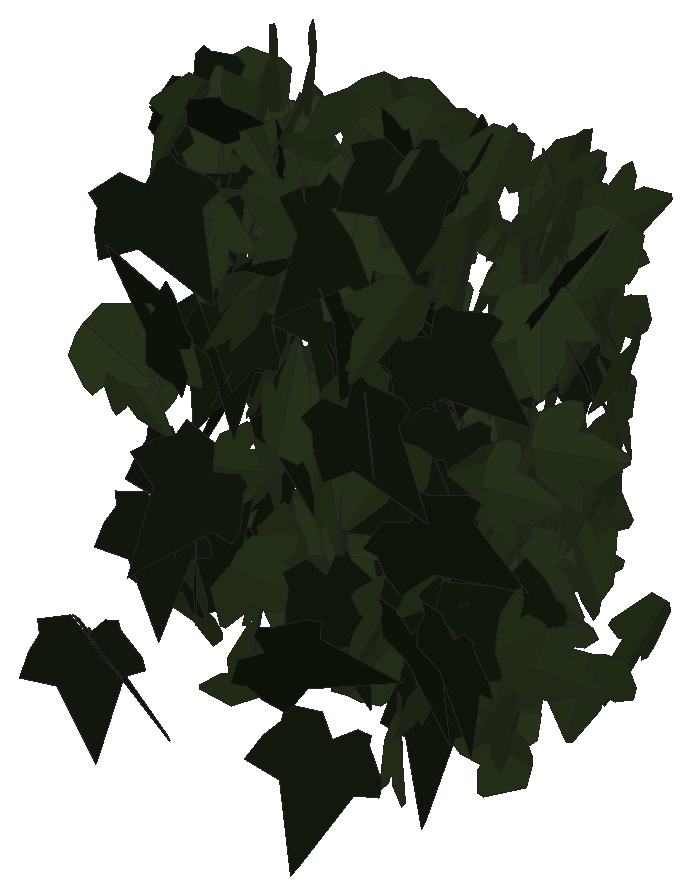
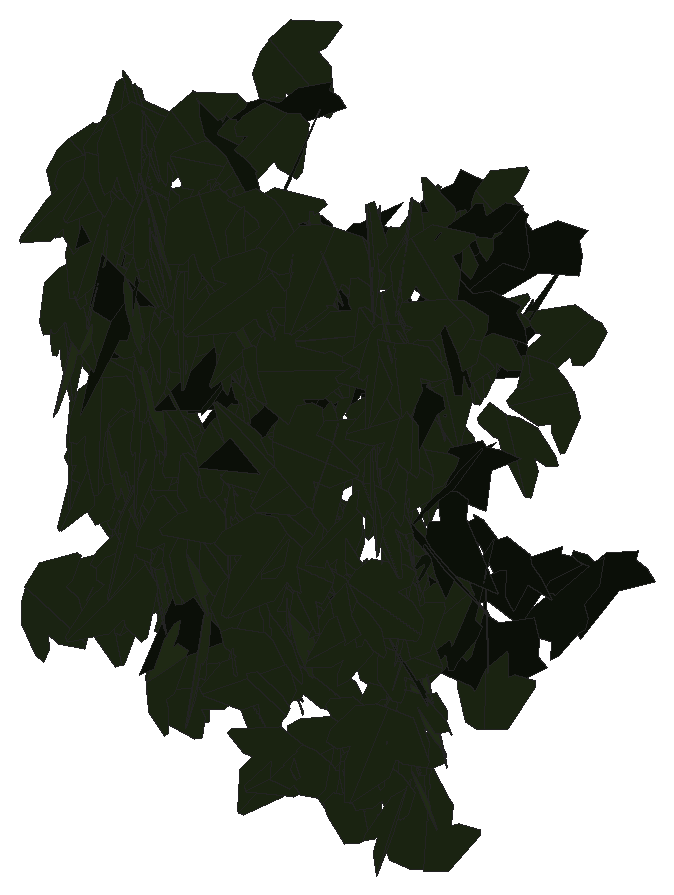
# SketchUp Ruby script. Lengths in inches.
U = 1.inch
M = Sketchup.active_model
def pt(a) = Geom::Point3d.new(a.map { |v| v * U })
def face(e, loops, mat)
  f = e.add_face(loops[0].map { |a| pt(a) })
  loops[1..].each { |l| e.add_face(l.map { |a| pt(a) }).erase! }
  f.material = f.back_material = mat if mat
  f
end
# faces: each face lists its corners as indices into pts; further lists are holes
def faces(e, pts, list, mat = nil) = list.each { |f| face(e, (f[0].is_a?(Array) ? f : [f]).map { |l| l.map { |i| pts[i] } }, mat) }
# xy, xz, yz: faces in a plane at the given z, y or x. An outline is a flat list of corners, or four numbers for a rectangle; further outlines are holes
def ring(l) = l.size == 4 ? [[l[0], l[1]], [l[2], l[1]], [l[2], l[3]], [l[0], l[3]]] : l.each_slice(2).to_a
def flat(e, list, mat, &to3) = list.each { |f| face(e, (f[0].is_a?(Array) ? f : [f]).map { |l| ring(l).map { |u, v| to3.(u, v) } }, mat) }
def xy(e, z, list, mat = nil) = flat(e, list, mat) { |x, y| [x, y, z] }
def xz(e, y, list, mat = nil) = flat(e, list, mat) { |x, z| [x, y, z] }
def yz(e, x, list, mat = nil) = flat(e, list, mat) { |y, z| [x, y, z] }
def lines(e, pts, list) = list.each { |a, b| e.add_line(pt(pts[a]), pt(pts[b])) }
# prism: a flat outline (further loops are holes) pulled along v
def prism(e, loops, v, mat = nil)
  f = face(e, loops, mat); d = Geom::Vector3d.new(v.map { |x| x * U })
  f.pushpull(f.normal.samedirection?(d) ? d.length : -d.length)
end
def box(e, o, s, mat = nil) = prism(e, [[o, [o[0] + s[0], o[1], o[2]], [o[0] + s[0], o[1] + s[1], o[2]], [o[0], o[1] + s[1], o[2]]]], [0, 0, s[2]], mat)
def at(x, y, z, deg = 0) = Geom::Transformation.translation(pt([x, y, z])) * Geom::Transformation.rotation(ORIGIN, Z_AXIS, deg.degrees)
def axes(o, x, y, z) = Geom::Transformation.new([*x, 0, *y, 0, *z, 0, *pt(o).to_a, 1])
def part(name) = M.definitions.add(name)
# library, detail: a bought-in or finely detailed component or shape, given as its bounding box
def library(name, o, s) = part(name).tap { |d| box(d.entities, o, s) }
def detail(e, o, s) = box(e.add_group.entities, o, s)
def put(e, d, t, mat = nil) = e.add_instance(d, t).tap { |i| i.material = mat if mat }
def group(e, t, mat = nil) = e.add_group.tap { |g| g.transformation = t; g.material = mat if mat }.entities
root = M.entities
M.materials.add("efeu1").color = [18, 25, 13]
M.materials.add("efeu2").color = [43, 57, 29]
c1 = part("ivyleaf_9")
p = [[1.54,2.16,1.25],[1.36,2.04,1.19],[-0.21,0.99,0.68],[-0.71,1.11,0.82],[-0.85,0.86,0.67],[-0.8,0.17,0.21],
  [-0.9,-0.01,0.1],[-0.67,-0.16,-0.02],[-0.08,-0.08,-0.05],[-0.03,-0.6,-0.4],[0.65,-0.88,-0.66],[0.83,-0.6,-0.49],
  [1.29,-0.42,-0.43],[1.8125,-0.07,-0.26],[1.21,0.44,0.15]]
faces(c1.entities,p,[[0,1,2,3,4,5,6,7,8,9,10,11,12,13,14]],"efeu1")
c2 = part("ivyleaf_10")
p = [[0,0.5,-0.03],[-0.0625,2.02,-0.43],[-0.19,2.01,-0.46],[-0.54,1.05,-0.29],[-0.52,0.625,-0.18],[-0.83,0.76,-0.28],
  [-1.16,0.64,-0.33],[-1.15,0.33,-0.24],[-0.77,-0.39,0.02],[-0.3,-0.51,0.16],[0.04,-0.48,0.23],[-0.02,2.01,-0.4375],
  [-0.06,2.01,-0.43],[0.04,-0.49,0.23],[0.67,-0.49,0.14],[1.38,0.36,-0.2],[1.375,0.51,-0.24],[0.81,0.65,-0.19],
  [0.62,0.59,-0.15],[0.6,1.09,-0.28],[0.5,1.23,-0.31]]
faces(c2.entities,p,[[0,1,2,3,4,5,6,7,8,9,10],[11,12,0,13,14,15,16,17,18,19,20]],"efeu2")
put(root,c1,axes([9.17,224.05,214.04],[0.13426,-0.23577,-0.35753],[-0.09997,0.33417,-0.27316],[0.43897,0.14822,0.04715]))
put(root,c2,axes([9.24,223.43,211.11],[0.46615,-0.05316,0.0105],[0.01092,-0.00051,-0.45228],[0.05741,0.43174,0.00076]))
put(root,c2,axes([9.23,225.49,212.94],[0.42615,0.1831,0.00128],[0.00474,-0.00653,-0.45233],[-0.19769,0.39453,-0.00808]))
put(root,c2,axes([9.27,225.45,207.26],[-0.10387,0.42195,0.04576],[-0.00867,0.0433,-0.45008],[-0.45809,-0.09649,-0.00185]))
put(root,c2,axes([9.33,223.75,214.05],[0.02415,-0.35025,0.26727],[0.03853,-0.25498,-0.36465],[0.46759,0.03911,0.01624]))
put(root,c1,axes([9.625,224.9,210.46],[-0.40097,0.19649,0.11756],[-0.1057,0.05671,-0.43684],[-0.22082,-0.38393,-0.00436]))
put(root,c2,axes([9.32,223.92,212.64],[-0.12434,-0.41878,0.02536],[0.06862,-0.0424,-0.44537],[0.44782,-0.10978,0.07529]))
put(root,c1,axes([9.16,224.26,213.17],[-0.21371,-0.23332,-0.32161],[0.2612,0.19686,-0.31541],[0.32683,-0.30989,0.04178]))
put(root,c2,axes([9.55,225.67,209.93],[0.17728,0.24306,-0.3341],[-0.34746,-0.12966,-0.273],[-0.26183,0.33665,0.13607]))
put(root,c2,axes([9.13,224.94,207.97],[-0.02965,-0.17998,-0.41087],[0.22092,-0.35452,0.15319],[-0.41356,-0.17648,0.11129]))
put(root,c1,axes([9.38,224.49,210.33],[-0.23041,0.1658,-0.35455],[0.24939,-0.2534,-0.27846],[-0.32469,-0.31229,0.03771]))
put(root,c2,axes([9.4,224.86,213.875],[-0.18721,-0.33137,0.23109],[0.02394,-0.2499,-0.36958],[0.43022,-0.13028,0.12113]))
put(root,c2,axes([9.32,225.5,211.44],[-0.39378,0.22473,-0.07906],[0.06642,-0.04508,-0.44539],[-0.24746,-0.36971,0.00625]))
put(root,c2,axes([9.5,224.1875,212.34],[0.04797,0.27211,0.41672],[-0.11252,-0.40188,0.27538],[0.48481,-0.1202,0.02268]))
put(root,c2,axes([9.51,224.79,209.52],[-0.13322,0.16794,0.39712],[-0.22639,0.31931,-0.21648],[-0.3895,-0.24303,-0.01]))
put(root,c2,axes([9.22,225.29,209.31],[-0.38063,0.02239,0.26416],[0.2688,-0.06401,0.36501],[0.05988,0.42968,0.04062]))
put(root,c2,axes([9.4,224.81,206.39],[-0.3092,-0.3194,-0.07533],[-0.04238,-0.06206,0.44591],[-0.35116,0.28872,0.01251]))
put(root,c1,axes([9.35,224.45,208.75],[0.29851,-0.33407,0.03644],[-0.01285,0.03561,0.45071],[-0.36254,-0.27633,0.01402]))
put(root,c2,axes([9.375,225.55,213.04],[0.01099,-0.40739,-0.15825],[0.07348,0.15183,-0.418],[0.46389,-0.0144,0.06996]))
put(root,c1,axes([9.32,223.58,209.72],[-0.35009,-0.09176,-0.28619],[0.29077,0.05843,-0.3501],[0.11661,-0.42118,0.01378]))
put(root,c1,axes([9.24,224.35,212.29],[-0.01028,0.28264,0.41232],[0.00326,-0.41236,0.28275],[0.49988,0.00851,0.00664]))
put(root,c2,axes([9.39,225.09,211.97],[0.04685,-0.10832,0.48587],[-0.07944,0.48014,0.1147],[-0.49142,-0.08794,0.02778]))
put(root,c2,axes([9.47,224.41,212.23],[-0.11992,-0.41782,0.05014],[-0.01362,-0.04654,-0.44961],[0.45403,-0.11175,-0.00024]))
put(root,c2,axes([9.39,225.3125,209.08],[-0.02553,-0.22466,0.38662],[0.07744,-0.36921,-0.2273],[0.46267,0.0494,0.05938]))
put(root,c2,axes([9.37,225.61,208.26],[-0.3357,-0.26445,-0.15659],[0.13636,0.08376,-0.42407],[0.29903,-0.33507,0.01758]))
put(root,c2,axes([9.3,224.32,209.27],[-0.08532,-0.16737,-0.40941],[0.20956,0.34275,-0.19205],[0.41172,-0.20913,0.0129]))
put(root,c2,axes([9.24,225.08,207.45],[0.24712,-0.20349,0.32132],[0.23558,-0.21922,-0.31816],[0.32272,0.31585,-0.01381]))
put(root,c2,axes([9.26,224.59,212.91],[0.10918,0.25113,0.35412],[0.12528,0.32022,-0.28143],[-0.43943,0.15369,0.00775]))
put(root,c2,axes([9.45,225.57,211.44],[0.15298,-0.38595,-0.14783],[-0.00667,0.14832,-0.42524],[0.44415,0.13516,0.04453]))
put(root,c2,axes([9.35,223.74,207.74],[-0.46831,0.04056,0.1704],[0.1629,-0.07795,0.46625],[0.06439,0.49222,0.0598]))
put(root,c2,axes([9.25,225.24,210.54],[0.22533,-0.24928,0.30062],[0.24733,-0.18179,-0.33496],[0.3298,0.30665,0.0458]))
put(root,c1,axes([9.42,224.4,211.0625],[-0.26986,-0.35546,-0.0218],[0.0128,0.01728,-0.45187],[0.38435,-0.25015,-0.00025]))
put(root,c2,axes([9.38,224.52,211.24],[0.04604,-0.22024,0.38761],[-0.01851,0.37335,0.23148],[-0.46717,-0.0365,0.02903]))
put(root,c1,axes([9.36,223.68,213.89],[0.37588,0.2587,-0.03557],[-0.02557,-0.02548,-0.45095],[-0.28066,0.34878,-0.00656]))
put(root,c1,axes([9.27,224.52,210.88],[0.05012,-0.42276,0.09501],[0.00283,-0.09161,-0.44225],[0.46711,0.04591,-0.00752]))
put(root,c2,axes([9.2,224.36,212.67],[0.09736,0.07088,-0.4364],[0.34577,0.27127,0.11919],[0.30278,-0.33259,0.00421]))
put(root,c2,axes([9.5,225.5625,211.06],[0.42123,-0.15778,-0.11493],[-0.10337,0.05782,-0.4372],[0.18054,0.40123,0.01781]))
put(root,c2,axes([9.46,224.03,213.3125],[0.13888,0.40062,-0.11484],[0.03148,0.10661,0.43755],[0.4477,-0.13177,0.00486]))
put(root,c2,axes([9.36,223.93,212.46],[0.45661,0.09135,0.04802],[0.03968,0.0477,-0.44804],[-0.10318,0.42262,0.04019]))
put(root,c1,axes([9.55,225.09,208.98],[-0.40007,0.11937,-0.20207],[0.19584,-0.07057,-0.40462],[-0.14934,-0.41231,0.01075]))
put(root,c2,axes([9.46,225.17,208.34],[0.46323,0.02487,-0.07084],[-0.07418,0.00828,-0.44664],[-0.02511,0.43421,0.01257]))
put(root,c2,axes([9.45,225.32,211.96],[-0.42649,0.16986,-0.06919],[0.0666,-0.02498,-0.44708],[-0.18542,-0.39968,-0.00146]))
put(root,c1,axes([9.375,223.17,209.14],[-0.09583,-0.41897,-0.07933],[0.01537,0.07496,-0.44539],[0.45967,-0.08985,-0.00165]))
put(root,c2,axes([9.34,222.19,211.78],[0.12877,0.28798,0.31558],[0.13339,0.27723,-0.3241],[-0.43167,0.17157,-0.00601]))
put(root,c2,axes([9.4375,225.07,208.22],[0.25243,0.36683,-0.00573],[0.0012,-0.00724,-0.45234],[-0.39622,0.23368,-0.00502]))
put(root,c2,axes([9.26,222.64,211.1875],[-0.24997,0.05642,-0.37853],[0.35206,-0.16872,-0.24278],[-0.18516,-0.39696,0.04939]))
put(root,c2,axes([9.56,225.19,213.1875],[0.17855,-0.40216,-0.01308],[-0.00422,0.01199,-0.45221],[0.43453,0.16537,0.00098]))
put(root,c2,axes([9.45,225.31,211.9375],[-0.43379,0.07735,-0.15394],[0.15104,-0.05497,-0.42455],[-0.0986,-0.42452,0.02692]))
put(root,c2,axes([9.45,225.16,207.8],[0.33395,0.30555,0.01637],[0.01216,0.01099,-0.4521],[-0.33021,0.30942,-0.0001]))
put(root,c2,axes([9.61,224.47,212.32],[0.20966,-0.38427,-0.06475],[-0.03794,0.052,-0.44767],[0.41871,0.19712,-0.00814]))
put(root,c1,axes([9.39,223.58,208.13],[-0.21274,-0.03123,0.40205],[0.41821,-0.04025,0.20182],[0.02359,0.43201,0.04787]))
put(root,c1,axes([9.375,223.75,208.94],[-0.05298,-0.02352,-0.44885],[0.44437,-0.13557,-0.04096],[-0.14296,-0.41267,0.03903]))
put(root,c1,axes([9.4,222.9375,213.29],[-0.05157,-0.31318,-0.38634],[0.11431,0.37055,-0.31564],[0.48402,-0.12088,0.03338]))
put(root,c2,axes([9.65,224.42,211.36],[-0.02962,-0.49129,-0.08806],[0.01275,0.08745,-0.49213],[0.49896,-0.0314,0.00734]))
put(root,c2,axes([9.63,224.91,210.34],[0.02736,-0.40702,-0.15743],[0.02014,0.15252,-0.42324],[0.46857,0.01721,0.02738]))
put(root,c2,axes([9.64,224.71,214.125],[0.17981,-0.36393,-0.29192],[-0.01136,0.30935,-0.39265],[0.46641,0.14784,0.10298]))
put(root,c2,axes([9.28,225.08,211.34],[-0.03612,0.00945,-0.45095],[0.39052,-0.23955,-0.03443],[-0.25866,-0.36298,0.01098]))
put(root,c2,axes([9.54,225.16,208.49],[-0.20583,0.26462,0.2994],[0.18509,-0.23133,0.33914],[0.37959,0.25629,-0.00302]))
put(root,c2,axes([9.46,225.1,212.49],[0.39764,0.20222,-0.2258],[0.18967,0.12455,0.44555],[0.23645,-0.43999,0.02234]))
put(root,c1,axes([9.35,224.9,212.23],[0.48622,-0.10323,0.05416],[0.05292,-0.01154,-0.49706],[0.10387,0.48909,-0.0003]))
put(root,c2,axes([9.31,225.28,210.99],[0.13091,-0.12269,0.4667],[0.44463,-0.15725,-0.16606],[0.18752,0.4585,0.06793]))
put(root,c2,axes([9.72,225.48,209.33],[0.04662,-0.04156,0.49608],[-0.12252,0.48197,0.05189],[-0.48251,-0.12639,0.03476]))
put(root,c1,axes([9.46,225.03,209.66],[0.23224,-0.37535,0.04759],[0.02647,-0.0387,-0.44989],[0.40752,0.21642,0.0021]))
put(root,c1,axes([9.84,222.86,211.57],[0.07403,-0.4705,0.15216],[-0.02373,0.1503,0.47629],[-0.49392,-0.07774,-0.00008]))
put(root,c1,axes([9.62,221.61,208.42],[-0.15044,-0.37027,-0.18814],[0.05184,0.17508,-0.41112],[0.44203,-0.14655,-0.01581]))
put(root,c2,axes([9.47,225.43,207.56],[0.32307,0.0626,0.32194],[0.31939,0.09412,-0.317],[-0.11971,0.42006,0.02305]))
put(root,c2,axes([9.53,225.81,209.78],[0.37364,-0.07058,0.26423],[0.26841,-0.0528,-0.36721],[0.09519,0.42597,-0.00174]))
put(root,c1,axes([9.46,221.98,208.19],[0.34901,-0.26872,0.11669],[0.09702,-0.06743,-0.43706],[0.29915,0.33536,0.00562]))
put(root,c2,axes([10.125,224.63,212.37],[-0.16838,-0.09001,-0.46211],[-0.41499,-0.2034,0.19082],[-0.22234,0.4478,-0.00621]))
put(root,c2,axes([9.6875,225.48,208.07],[-0.36731,0.1028,-0.26102],[0.22296,-0.16293,-0.36035],[-0.18996,-0.39001,0.08174]))
put(root,c2,axes([9.64,225.22,211.54],[0.10424,-0.25481,0.41738],[0.3017,-0.30234,-0.25993],[0.38485,0.30604,0.09072]))
put(root,c2,axes([9.49,224.17,213.78],[0.23592,-0.00784,0.44077],[0.44084,0.00453,-0.23588],[-0.0003,0.49992,0.00905]))
put(root,c2,axes([9.91,225.08,214.125],[0.23244,-0.39917,-0.1914],[-0.03567,0.19859,-0.45748],[0.44125,0.22633,0.06384]))
put(root,c1,axes([9.79,224.88,212.49],[-0.03425,-0.01446,0.49862],[0.01013,-0.49971,-0.01379],[0.49872,0.00916,0.03452]))
put(root,c2,axes([9.97,225.32,210.52],[0.08143,-0.01875,-0.49297],[0.03997,0.49825,-0.01234],[0.4917,-0.0374,0.08265]))
put(root,c2,axes([9.9,225.29,206.83],[0.09448,-0.48658,-0.06567],[0.022,-0.06262,0.49558],[-0.4905,-0.09653,0.00958]))
put(root,c2,axes([9.77,225.34,211.58],[0.31412,0.21991,0.2467],[0.20348,0.14413,-0.37921],[-0.28397,0.34654,0.00116]))
put(root,c2,axes([9.7,225.1,209.41],[0.15077,-0.07794,-0.47031],[0.46048,-0.10389,0.16483],[-0.12341,-0.48284,0.04045]))
put(root,c2,axes([9.79,225.08,212.85],[0.12007,-0.05897,0.43305],[0.32772,0.30946,-0.03869],[-0.31448,0.29997,0.12503]))
put(root,c1,axes([9.88,224.58,211.93],[-0.18931,-0.39806,0.00711],[0.42466,-0.17426,-0.06776],[0.06735,-0.02007,0.44724]))
put(root,c2,axes([10.49,225.74,211.47],[-0.00597,0.02453,-0.49936],[-0.4709,0.16752,0.01386],[0.16799,0.47046,0.0211]))
put(root,c2,axes([10.12,224.44,208.24],[-0.48238,-0.12794,0.03069],[0.04198,-0.03915,0.49669],[-0.12469,0.48177,0.04851]))
put(root,c2,axes([10.43,225.58,209.89],[-0.09571,0.12749,-0.47391],[-0.32239,0.3477,0.15865],[0.37,0.33594,0.01564]))
put(root,c2,axes([10.16,225.54,211.59],[-0.26854,0.39612,-0.14481],[0.08066,-0.12027,-0.47857],[-0.41398,-0.2804,0.00069]))
put(root,c2,axes([10.63,225.49,210.41],[0.24965,-0.03764,-0.43158],[-0.42662,0.0652,-0.25247],[0.07528,0.4943,0.00044]))
put(root,c2,axes([10.8125,225.62,212.27],[-0.12604,0.12606,-0.46714],[-0.48289,-0.00237,0.12965],[0.03048,0.48384,0.12235]))
put(root,c2,axes([10.43,225.24,213.74],[-0.3137,-0.33861,-0.19217],[0.14942,0.12319,-0.46098],[0.35953,-0.34665,0.0239]))
put(root,c2,axes([10.43,224.83,209.27],[-0.06239,0.49353,-0.05039],[0.00544,-0.05011,-0.49745],[-0.49606,-0.06262,0.00089]))
put(root,c2,axes([10.59,225.35,212.8125],[0.46416,0.10744,-0.1517],[-0.15022,-0.02358,-0.47632],[-0.1095,0.48775,0.01039]))
put(root,c2,axes([10.33,225.58,211.2],[-0.37182,0.03772,-0.33216],[0.32998,-0.03811,-0.37371],[-0.05351,-0.49712,0.00344]))
put(root,c2,axes([10.58,223.92,212.93],[-0.0979,0.34101,0.35232],[0.0733,-0.34505,0.35435],[0.48481,0.12103,0.01757]))
put(root,c2,axes([10.82,225.375,211.24],[0.31679,-0.12792,-0.36507],[-0.3398,0.1335,-0.34164],[0.18488,0.46456,-0.00235]))
put(root,c2,axes([10.45,223.31,208.81],[-0.17558,-0.24536,-0.39871],[0.27437,0.29111,-0.29996],[0.37933,-0.32412,0.03241]))
put(root,c2,axes([10.42,225.18,207.42],[-0.11155,-0.11661,-0.47324],[0.31749,0.35097,-0.16131],[0.36981,-0.33649,-0.00426]))
put(root,c2,axes([10.51,224.875,209.91],[0.02874,0.04497,0.49714],[0.06406,0.49352,-0.04834],[-0.49505,0.06647,0.0226]))
put(root,c2,axes([10.62,224.32,212.66],[-0.33267,0.28023,0.24658],[0.17059,-0.17964,0.43431],[0.332,0.3731,0.02392]))
put(root,c2,axes([10.86,224.3,211.63],[0.09859,-0.14269,0.46896],[-0.27671,0.37864,0.17338],[-0.40461,-0.29372,-0.00431]))
put(root,c2,axes([10.65,223.71,210.43],[0.48147,-0.13432,0.012],[-0.00983,0.00942,0.49981],[-0.13449,-0.48153,0.00643]))
put(root,c2,axes([10.91,225.05,208.29],[0.34712,0.10055,-0.34554],[-0.33035,-0.10137,-0.36137],[-0.14273,0.47918,-0.00394]))
put(root,c2,axes([10.57,225.52,209.16],[0.18764,-0.26669,0.37903],[0.23791,-0.2955,-0.3257],[0.39773,0.30258,0.016]))
put(root,c2,axes([10.69,225.01,213.57],[0.35609,-0.31025,0.16417],[0.117,-0.11556,-0.47218],[0.33093,0.37469,-0.0097]))
put(root,c2,axes([10.5625,225.68,207.52],[0.32362,0.23482,0.30022],[0.23426,0.18813,-0.39966],[-0.30066,0.39933,0.01174]))
put(root,c2,axes([10.83,225.59,210.05],[-0.40981,-0.16239,-0.23598],[0.21502,0.09777,-0.44069],[0.18927,-0.46268,-0.0103]))
put(root,c1,axes([11,221.98,210.77],[-0.26137,-0.38705,0.17853],[-0.09975,-0.14807,-0.46704],[0.41441,-0.27976,0.00018]))
put(root,c2,axes([10.75,224.63,209.21],[-0.03918,0.04455,-0.49647],[0.18716,-0.46025,-0.05607],[-0.46199,-0.19023,0.01939]))
put(root,c2,axes([11.19,225.57,207.99],[0.32489,-0.17434,-0.33772],[-0.30044,0.1543,-0.36868],[0.23277,0.44249,-0.0045]))
put(root,c2,axes([10.93,225.43,211.96],[-0.00355,-0.44485,-0.22825],[0.06456,-0.22676,0.44092],[-0.4958,-0.02634,0.05905]))
put(root,c2,axes([10.86,225.6,209],[0.40559,-0.19217,0.22039],[0.20865,-0.07381,-0.44835],[0.20485,0.45566,0.02032]))
put(root,c2,axes([11.12,225.07,212.91],[0.07562,-0.44922,0.20612],[0.01793,-0.20589,-0.45529],[0.49392,0.07625,-0.01503]))
put(root,c2,axes([11.04,224.83,212.36],[-0.35903,-0.19573,-0.28773],[0.25065,0.14133,-0.4089],[0.2414,-0.43785,-0.00336]))
put(root,c1,axes([11.03,224.71,211.04],[0.23785,0.20645,0.38834],[0.26531,0.28476,-0.31388],[-0.35077,0.35537,0.02592]))
put(root,c1,axes([11.21,224.09,212.93],[-0.182,-0.37966,0.26969],[-0.09115,-0.25492,-0.42037],[0.45669,-0.20218,0.02358]))
put(root,c2,axes([10.9375,225.625,208.45],[-0.29165,0.05766,-0.40201],[0.39623,-0.06821,-0.29724],[-0.08912,-0.49196,-0.00591]))
put(root,c2,axes([11.08,225.43,213.9],[-0.42164,0.12855,-0.236],[0.22025,-0.08632,-0.4405],[-0.15399,-0.47542,0.01617]))
put(root,c2,axes([10.95,225.48,210.87],[0.37572,-0.02833,-0.32868],[0.32979,0.01939,0.37532],[-0.00852,-0.49882,0.03326]))
put(root,c2,axes([11.34,225.23,213.78],[-0.22783,-0.36848,0.24963],[-0.03747,-0.26357,-0.42324],[0.4435,-0.21156,0.09249]))
put(root,c2,axes([11.09,225.52,213.24],[-0.18141,-0.20163,-0.42004],[0.31099,0.28326,-0.27028],[0.34695,-0.35932,0.02263]))
put(root,c1,axes([11.1,223.89,208.67],[0.13053,-0.44108,-0.196],[-0.05949,0.18679,-0.45997],[0.47898,0.14339,-0.00371]))
put(root,c2,axes([11.28,224.06,212.91],[0.46648,0.16986,-0.05953],[-0.05741,-0.01632,-0.49642],[-0.17059,0.46998,0.00428]))
put(root,c2,axes([11.3,225.09,212.54],[0.00604,0.29082,0.40668],[0.01089,0.40654,-0.29088],[-0.49984,0.01237,-0.00142]))
put(root,c1,axes([11.35,224.03,212.125],[-0.30908,-0.35942,-0.15901],[0.10179,0.12219,-0.47404],[0.37962,-0.3254,-0.00236]))
put(root,c2,axes([11.66,224.74,209.22],[0.30393,0.0049,-0.39699],[-0.39698,0.01081,-0.30379],[0.00561,0.49986,0.01046]))
put(root,c2,axes([11.375,225.37,208.57],[-0.0278,-0.17828,0.46631],[0.10609,-0.45847,-0.16896],[0.48782,0.08954,0.06332]))
put(root,c2,axes([11.69,225.05,208.92],[-0.21177,-0.25999,0.37089],[-0.20919,-0.307,-0.33465],[0.40174,-0.29691,0.02125]))
put(root,c2,axes([11.49,224.8,213.24],[0.15129,-0.46438,0.10706],[0.02737,-0.10367,-0.48837],[0.47578,0.15363,-0.00595]))
put(root,c2,axes([11.59,224.33,208.51],[0.13207,-0.40388,-0.26351],[-0.08229,0.25033,-0.42493],[0.47517,0.1556,-0.00035]))
put(root,c1,axes([11.32,224.62,211.47],[0.48962,-0.06341,-0.07904],[-0.07776,0.01499,-0.49369],[0.06498,0.49574,0.00482]))
put(root,c2,axes([11.56,225.01,211.22],[-0.07741,-0.39665,0.29441],[0.06444,-0.30356,-0.39204],[0.48975,-0.02275,0.09812]))
put(root,c2,axes([11.64,224.95,213.21],[-0.19961,-0.45754,0.0286],[-0.00949,-0.02707,-0.49918],[0.45833,-0.19982,0.00212]))
put(root,c1,axes([11.18,224.1,211.75],[0.08577,-0.11271,-0.47952],[0.42953,0.25539,0.0168],[0.24114,-0.41482,0.14063]))
put(root,c1,axes([11.8,224.88,213.08],[0.00383,0.01855,-0.49964],[-0.15317,-0.47559,-0.01884],[-0.47595,0.1532,0.00204]))
put(root,c1,axes([11.35,224.14,211.38],[0.27107,-0.41147,-0.08492],[-0.03858,0.07625,-0.49264],[0.41837,0.27363,0.00959]))
put(root,c1,axes([11.41,223.98,211.84],[0.04236,-0.31391,0.38687],[0.04032,-0.38483,-0.31667],[0.49657,0.05803,-0.00729]))
put(root,c2,axes([11.46,225.49,212.86],[0.17314,-0.23227,0.40752],[0.24742,-0.32383,-0.28969],[0.39851,0.30197,0.0028]))
put(root,c2,axes([11.73,225.4,210.95],[-0.05345,-0.43868,0.23389],[-0.01759,-0.23342,-0.44182],[0.49682,-0.05546,0.00952]))
put(root,c2,axes([11.78,225.19,210.77],[-0.145,-0.47265,0.07468],[-0.01768,-0.07269,-0.49437],[0.47819,-0.14601,0.00437]))
put(root,c2,axes([11.97,225.47,213.7],[-0.42074,-0.11229,0.2457],[-0.23682,-0.06547,-0.43546],[0.12997,-0.48281,0.00191]))
put(root,c2,axes([11.8125,225.23,210.31],[0.26014,-0.34554,-0.25085],[-0.07334,0.25322,-0.42485],[0.42065,0.25784,0.08107]))
put(root,c1,axes([11.67,224.6,213.47],[-0.10576,-0.09037,0.48026],[-0.03745,-0.48843,-0.10015],[0.48725,-0.05715,0.09654]))
put(root,c2,axes([11.65,223.87,207.65],[-0.09201,-0.39968,0.28599],[0.06715,0.27801,0.41012],[-0.48685,0.11388,0.00252]))
put(root,c2,axes([11.8,225.15,212.54],[0.05138,-0.49728,-0.00839],[0.00092,0.00853,-0.49993],[0.49735,0.05135,0.00179]))
put(root,c2,axes([11.79,223.44,211.64],[-0.14255,-0.35463,-0.32236],[0.10494,0.30506,-0.38201],[0.46762,-0.17657,-0.01254]))
put(root,c2,axes([11.87,225.57,208.49],[0.22819,-0.27831,-0.34709],[-0.0431,0.37442,-0.32856],[0.4428,0.17987,0.14689]))
put(root,c2,axes([11.73,225.19,212.66],[-0.03077,-0.12962,-0.48193],[0.12547,-0.46934,0.11822],[-0.48302,-0.11365,0.06141]))
put(root,c2,axes([11.72,225.38,209.99],[0.35171,0.258,-0.24441],[0.19959,0.14112,0.43617],[0.29405,-0.40438,-0.00372]))
put(root,c2,axes([11.56,225.27,211.66],[0.07929,-0.11117,0.48099],[0.44073,-0.20355,-0.1197],[0.22242,0.44296,0.06572]))
put(root,c2,axes([11.84,223.97,208.62],[0.06993,-0.30339,0.39123],[0.12235,-0.37227,-0.31055],[0.47973,0.13917,0.02217]))
put(root,c1,axes([11.62,224.3,210.49],[0.35236,-0.15617,-0.31852],[0.29079,-0.12999,0.38542],[-0.20319,-0.45685,-0.00078]))
put(root,c2,axes([11.85,225.16,212.15],[0.07726,-0.35066,0.34795],[0.20694,-0.29681,-0.34508],[0.44856,0.19733,0.09927]))
put(root,c1,axes([11.68,224.61,211.66],[0.44505,0.0815,0.21281],[0.20734,0.04892,-0.45235],[-0.09456,0.49088,0.00975]))
put(root,c2,axes([11.78,225.12,210.61],[0.30916,-0.21197,0.3309],[0.29076,-0.15983,-0.37405],[0.26435,0.4237,0.02444]))
put(root,c2,axes([12.28,223.53,210.75],[-0.26967,-0.32954,0.26207],[-0.13271,-0.22883,-0.42429],[0.39959,-0.29839,0.03595]))
put(root,c1,axes([12.09,222.68,207.54],[-0.30713,-0.38365,-0.0921],[0.05554,0.07352,-0.49144],[0.39063,-0.3121,-0.00254]))
put(root,c2,axes([11.99,224.88,213.37],[0.12384,0.41835,0.24422],[0.0674,0.23474,-0.43629],[-0.47971,0.14098,0.00175]))
put(root,c2,axes([12.26,225.1,209.35],[-0.1516,-0.40234,0.25522],[-0.08149,-0.24199,-0.42988],[0.46945,-0.17193,0.0078]))
put(root,c2,axes([12.52,224.65,208.75],[0.13939,0.02532,-0.47951],[-0.47741,0.06086,-0.13557],[0.0515,0.49564,0.04114]))
put(root,c1,axes([12.01,223.45,211.09],[-0.05222,0.06655,0.49279],[0.05695,-0.49144,0.0724],[0.49399,0.06369,0.04375]))
put(root,c1,axes([12.06,224.125,210.08],[-0.23417,-0.31285,-0.31192],[0.17788,0.25638,-0.39068],[0.40438,-0.29394,-0.00878]))
put(root,c2,axes([12.26,224.41,213.2],[0.20028,-0.45497,-0.05378],[-0.01744,0.05108,-0.49708],[0.4578,0.20098,0.00459]))
put(root,c1,axes([12.02,225.01,211.43],[-0.00212,-0.37618,0.32937],[0.13838,-0.31695,-0.3611],[0.48047,0.08963,0.10545]))
put(root,c2,axes([12.07,225.48,209.36],[0.22465,-0.25263,0.36839],[0.25708,-0.2641,-0.33788],[0.3653,0.34122,0.01123]))
put(root,c1,axes([12.21,224.7,210.49],[-0.09155,-0.48885,0.05146],[-0.00883,-0.0507,-0.49734],[0.49147,-0.09197,0.00065]))
put(root,c2,axes([12.4,225.21,212.46],[0.10986,-0.44479,-0.20023],[-0.01352,0.20239,-0.45701],[0.48759,0.10583,0.03244]))
put(root,c2,axes([12.65,225.39,207.65],[-0.18232,0.28434,-0.36866],[-0.26219,0.26446,0.33364],[0.38473,0.31498,0.05267]))
put(root,c2,axes([12.11,223.77,207.25],[0.15267,-0.07313,0.47047],[0.3987,-0.25042,-0.16831],[0.26025,0.42655,-0.01815]))
put(root,c1,axes([12.71,224.17,214.02],[-0.25449,0.39274,0.17604],[-0.09466,0.14843,-0.46798],[-0.41985,-0.27152,-0.0012]))
put(root,c1,axes([12.28,223.74,214.26],[-0.07865,-0.46045,-0.17834],[0.06328,0.1697,-0.46605],[0.4897,-0.09588,0.03158]))
put(root,c2,axes([12.48,223.92,207.9],[-0.02671,-0.41341,-0.27997],[0.00815,0.27997,-0.41419],[0.49922,-0.02669,-0.00822]))
put(root,c2,axes([12.31,223.72,213.98],[-0.08821,-0.30097,-0.3894],[0.23854,0.31989,-0.30128],[0.43048,-0.23893,0.08715]))
put(root,c2,axes([12.48,224.75,213.25],[0.1535,-0.47388,-0.0433],[-0.01326,0.04122,-0.49812],[0.47567,0.15407,0.00009]))
put(root,c2,axes([12.51,225.02,209.59],[-0.34329,-0.35998,-0.05065],[0.03445,0.03714,-0.49743],[0.36189,-0.34501,-0.0007]))
put(root,c1,axes([12.49,224.09,208.66],[-0.40632,-0.04997,0.28707],[0.28424,0.04043,0.40935],[-0.06412,0.49585,-0.00445]))
put(root,c1,axes([12.18,221.55,209.17],[0.0625,0.1625,-0.46871],[0.19848,0.42476,0.17373],[0.45464,-0.20778,-0.01142]))
put(root,c1,axes([12.41,224.07,207.68],[-0.35453,-0.08631,-0.34185],[0.33525,0.06755,-0.36475],[0.10915,-0.48784,0.00997]))
put(root,c2,axes([12.74,225.19,211.41],[0.06546,0.14434,0.47422],[-0.23123,-0.41421,0.15799],[0.43846,-0.23999,0.01253]))
put(root,c2,axes([12.87,224.9,207.24],[-0.0307,-0.02212,-0.49857],[-0.46352,-0.18385,0.0367],[-0.18495,0.46445,-0.00922]))
put(root,c2,axes([12.54,224.12,209.2],[-0.18962,-0.41825,-0.19776],[0.09788,0.17263,-0.45893],[0.45218,-0.21276,0.01641]))
put(root,c2,axes([12.42,224.61,209.59],[-0.29097,-0.21706,-0.34383],[0.26295,0.22204,-0.3627],[0.31015,-0.39189,-0.01506]))
put(root,c1,axes([12.48,224.26,208.4],[0.3808,0.2914,0.14168],[0.10943,0.09012,-0.47948],[-0.30498,0.39619,0.00486]))
put(root,c2,axes([12.64,224.36,213.64],[0.05672,0.24371,-0.43289],[0.08425,0.42467,0.25012],[0.48958,-0.10131,0.00711]))
put(root,c2,axes([12.66,224.43,208.06],[-0.3683,-0.30746,-0.14079],[0.10707,0.09144,-0.47977],[0.32076,-0.38355,-0.00152]))
put(root,c1,axes([12.3,224.25,208.65],[0.25764,-0.05646,0.42478],[0.41572,-0.08726,-0.26375],[0.10392,0.48908,0.00198]))
put(root,c1,axes([12.45,223.65,208.54],[0.18953,-0.40206,0.22897],[0.12543,-0.19352,-0.44364],[0.44536,0.22561,0.0275]))
put(root,c2,axes([12.44,225.28,210.68],[0.07146,-0.05862,-0.49138],[0.37411,-0.3186,0.09241],[-0.32394,-0.38087,-0.00168]))
put(root,c2,axes([12.87,225.21,211.83],[-0.48146,0.11362,0.07275],[-0.07072,0.01705,-0.49468],[-0.11489,-0.48662,-0.00035]))
put(root,c1,axes([12.5,222.52,211.83],[-0.06776,-0.14058,-0.47502],[0.37675,0.29669,-0.14154],[0.32166,-0.37712,0.06572]))
put(root,c2,axes([12.86,224.7,214.2],[-0.10678,-0.40084,0.27915],[0.04357,-0.29242,-0.40323],[0.48652,-0.06179,0.09738]))
put(root,c2,axes([12.81,225.06,211.86],[0.07003,-0.40636,0.28278],[0.10807,-0.26616,-0.40924],[0.48313,0.11844,0.05055]))
put(root,c2,axes([12.9,225.2,209.6],[0.46604,0.09169,-0.15619],[-0.15447,-0.02391,-0.47494],[-0.09456,0.49094,0.00604]))
put(root,c2,axes([12.92,225.29,210.71],[0.0901,-0.40869,-0.27359],[-0.03219,0.27265,-0.41788],[0.49076,0.09292,0.02282]))
put(root,c2,axes([12.9,225.15,213.22],[0.0311,-0.49893,-0.01021],[-0.00063,0.01019,-0.4999],[0.49903,0.03111,0]))
put(root,c2,axes([12.9375,225.47,209.63],[0.07596,-0.3064,-0.38775],[-0.01694,0.39046,-0.31186],[0.49391,0.06052,0.04893]))
put(root,c1,axes([12.67,223.4375,210.09],[-0.01988,-0.02523,-0.49897],[0.15363,0.47486,-0.03013],[0.4754,-0.15451,-0.01113]))
put(root,c2,axes([13.2,224.9,212.82],[-0.30546,-0.1067,-0.3812],[-0.36336,-0.11546,0.32348],[-0.15706,0.47464,-0.00701]))
put(root,c2,axes([13.29,224.25,207.13],[-0.12211,0.07352,-0.47925],[-0.48065,0.04663,0.12961],[0.06375,0.49236,0.05929]))
put(root,c2,axes([13,225.3125,210.5625],[-0.17852,-0.45865,0.08816],[-0.01211,-0.08981,-0.49172],[0.46689,-0.1777,0.02095]))
put(root,c2,axes([12.73,225.3,210.82],[0.08104,-0.22759,-0.43776],[0.20537,-0.38781,0.23964],[-0.44862,-0.21864,0.03062]))
put(root,c2,axes([13.09,225.28,209.67],[0.01917,0.10023,-0.48948],[-0.12121,0.47614,0.09275],[0.48471,0.11511,0.04255]))
put(root,c2,axes([12.9375,225.04,212.8125],[0.41936,-0.27149,0.02063],[-0.01076,0.02132,0.49943],[-0.27206,-0.41933,0.01204]))
put(root,c2,axes([12.94,225.51,208.82],[-0.07941,-0.19609,-0.45304],[0.17242,0.41894,-0.21156],[0.46256,-0.18983,0.00108]))
put(root,c2,axes([13.08,223.77,213.74],[-0.01268,-0.49848,-0.03689],[0.00448,0.03678,-0.49863],[0.49982,-0.01298,0.00353]))
put(root,c2,axes([13.13,224.78,210.03],[-0.17167,-0.45474,0.11721],[-0.04047,-0.11001,-0.48607],[0.46786,-0.17637,0.00097]))
put(root,c2,axes([13.125,224.88,208.7],[0.25384,-0.41055,-0.13043],[-0.06279,0.11451,-0.48264],[0.42617,0.26141,0.00658]))
put(root,c2,axes([13.11,225.52,210.47],[0.17452,-0.46653,0.04348],[0.01879,-0.03939,-0.49809],[0.46818,0.17549,0.00379]))
put(root,c1,axes([13.48,224.32,208.58],[-0.12373,0.03965,0.48282],[-0.47932,0.06229,-0.12795],[-0.0703,-0.49452,0.02259]))
put(root,c2,axes([12.95,224.48,211.65],[-0.34409,-0.25042,0.26248],[0.20944,0.15825,0.42555],[-0.29621,0.4028,-0.00401]))
put(root,c2,axes([13.44,225.1875,209.91],[-0.32071,-0.09539,0.37155],[-0.35958,-0.09392,-0.33449],[0.13361,-0.48175,-0.00835]))
put(root,c2,axes([13.08,224.8,210.33],[0.07104,-0.24523,0.4299],[0.12936,-0.41001,-0.25526],[0.47772,0.14749,0.00519]))
put(root,c2,axes([13.22,224.76,213.48],[0.04293,-0.20643,-0.45337],[-0.02362,0.45369,-0.20882],[0.49759,0.03935,0.0292]))
put(root,c2,axes([13.16,224.42,210.7],[-0.24083,0.43539,0.04939],[-0.02649,0.04179,-0.49755],[-0.43738,-0.24226,0.00294]))
put(root,c2,axes([13.15,225.18,212.23],[0.19541,-0.41613,0.19659],[0.09755,-0.17127,-0.45951],[0.44978,0.21794,0.01425]))
put(root,c2,axes([12.91,225.23,212.84],[0.24196,-0.14867,0.41152],[0.39775,-0.12125,-0.27766],[0.18235,0.46173,0.05959]))
put(root,c1,axes([13.03,223.3,212.54],[0.00191,-0.16991,-0.47024],[0.09823,0.46121,-0.16624],[0.49025,-0.09175,0.03514]))
put(root,c2,axes([13.19,224.85,213.16],[0.27325,-0.37753,0.18112],[0.09082,-0.15769,-0.46571],[0.40876,0.28741,-0.0176]))
put(root,c2,axes([13.31,224.26,210.79],[-0.05944,-0.09615,-0.48705],[-0.1333,-0.46943,0.10894],[-0.47822,0.1428,0.03017]))
put(root,c2,axes([13.33,225.21,214.125],[0.0122,-0.48894,0.10386],[0.02144,-0.10328,-0.48875],[0.49939,0.01638,0.01844]))
put(root,c1,axes([13.37,224.94,211.41],[-0.39591,-0.04349,0.30226],[0.30355,-0.00202,0.39731],[-0.03333,0.4981,0.028]))
put(root,c2,axes([13.4,224.58,208.6],[-0.43142,-0.21021,-0.1403],[0.13114,0.05107,-0.47978],[0.21604,-0.45078,0.01107]))
put(root,c1,axes([13.18,223.45,208.81],[0.14902,-0.43356,0.19954],[0.05729,-0.19128,-0.4584],[0.47383,0.15948,-0.00733]))
put(root,c1,axes([13.41,225.05,212.1],[0.37769,-0.10815,-0.30928],[-0.2962,0.08905,-0.39286],[0.14006,0.47997,0.0032]))
put(root,c2,axes([13.52,222.11,213.72],[-0.10238,-0.39122,0.29404],[-0.03178,-0.29446,-0.40284],[0.48837,-0.10118,0.03543]))
put(root,c2,axes([13.07,224.96,213.46],[-0.04501,-0.01115,0.49785],[0.49285,0.07048,0.04614],[-0.07121,0.49488,0.00464]))
put(root,c2,axes([13.57,223.98,208.03],[0.06646,-0.49343,-0.04598],[-0.01114,0.04489,-0.49786],[0.49544,0.06719,-0.00503]))
put(root,c2,axes([13.2,224.83,209.2],[-0.11813,0.02691,-0.4851],[0.40186,-0.27517,-0.11312],[-0.27305,-0.41661,0.04338]))
put(root,c2,axes([13.54,225.25,213.86],[0.05964,-0.38489,0.31353],[0.05963,-0.30794,-0.38938],[0.49284,0.08383,0.00917]))
put(root,c2,axes([13.5625,224.58,213.79],[0.28163,-0.41314,-0.00115],[-0.00164,0.00027,-0.5],[0.41314,0.28163,-0.0012]))
put(root,c2,axes([13.6,225.1875,210.69],[-0.10625,-0.47673,-0.10695],[0.02714,0.10352,-0.48841],[0.48783,-0.10959,0.00388]))
put(root,c2,axes([13.52,224.94,213.78],[-0.10507,-0.26692,-0.40953],[0.14803,0.38184,-0.28686],[0.46588,-0.18152,-0.00121]))
put(root,c2,axes([13.61,224.7,213.84],[0.03515,-0.4877,0.10446],[0.01632,-0.10354,-0.48889],[0.4985,0.03778,0.00864]))
put(root,c2,axes([13.28,224.85,213.875],[0.2135,-0.13189,0.43246],[0.41232,-0.13942,-0.24607],[0.1855,0.4617,0.04923]))
put(root,c2,axes([13.6,225.22,213.07],[-0.44656,-0.20155,-0.0998],[0.09211,0.03853,-0.48993],[0.20519,-0.45595,0.00272]))
put(root,c2,axes([13.48,224.66,214.11],[0.38914,-0.1859,0.253],[0.22927,-0.107,-0.43126],[0.21448,0.45166,0.00197]))
put(root,c2,axes([13.81,225.04,212.65],[-0.37459,0.26521,0.19836],[-0.16299,0.11308,-0.45896],[-0.2883,-0.40851,0.00174]))
put(root,c2,axes([13.77,225.41,212.21],[-0.1985,-0.45073,0.08628],[-0.02658,-0.08255,-0.49242],[0.45814,-0.20007,0.00881]))
put(root,c2,axes([13.7,225.11,210.05],[-0.07029,-0.3421,-0.35781],[0.07781,0.34927,-0.34922],[0.48888,-0.10478,0.00414]))
put(root,c2,axes([13.36,223.87,210.63],[0.03233,-0.01859,-0.49861],[0.47938,-0.13743,0.0362],[-0.13839,-0.48038,0.00893]))
put(root,c2,axes([13.83,225.03,212.47],[-0.02397,-0.46516,0.18179],[0.01611,-0.18262,-0.46518],[0.49917,-0.01644,0.02375]))
put(root,c2,axes([13.84,225.33,210.51],[0.1366,-0.41749,-0.23884],[-0.01808,0.24365,-0.43624],[0.48064,0.12782,0.05147]))
put(root,c2,axes([13.93,224.79,208.1875],[-0.38459,-0.296,0.1203],[-0.08332,-0.08884,-0.48494],[0.30846,-0.39306,0.01901]))
put(root,c2,axes([13.92,225.27,211.34],[0.2335,-0.0894,-0.433],[-0.10028,0.4662,-0.15034],[0.4306,0.15705,0.19978]))
put(root,c2,axes([14.1,224.75,209.31],[0.23665,-0.0431,0.43834],[-0.42011,0.12738,0.23933],[-0.1323,-0.48158,0.02407]))
put(root,c2,axes([13.8125,225.39,213.375],[0.0099,-0.10465,-0.48883],[0.09577,0.48026,-0.10088],[0.49064,-0.09164,0.02956]))
put(root,c2,axes([13.74,224.09,208.48],[-0.17775,-0.24911,-0.39541],[0.22451,0.32551,-0.306],[0.40988,-0.28633,-0.00386]))
put(root,c2,axes([13.74,224.2,212.8],[0.4789,0.12561,0.06982],[0.06406,0.03083,-0.49492],[-0.12864,0.48298,0.01344]))
put(root,c2,axes([13.58,223.91,208.72],[0.23536,-0.17675,-0.40418],[0.31068,-0.25882,0.29409],[-0.31318,-0.38958,-0.01201]))
put(root,c1,axes([13.96,224.17,213.08],[0.09116,0.36688,0.32724],[0.0826,0.31665,-0.37803],[-0.48463,0.12299,-0.00288]))
put(root,c2,axes([13.97,224.34,213.93],[0.05041,-0.39376,-0.30399],[-0.00822,0.30485,-0.39623],[0.49738,0.04495,0.02426]))
put(root,c2,axes([13.97,225.82,208.35],[0.06398,-0.37606,0.32324],[0.05079,-0.31924,-0.38145],[0.49328,0.08165,-0.00265]))
put(root,c2,axes([13.58,224.67,210.81],[0.07204,-0.04306,-0.49291],[0.48489,-0.09296,0.07899],[-0.09844,-0.48939,0.02836]))
put(root,c2,axes([14.01,225.33,211.78],[0.10567,-0.48112,-0.08577],[-0.00096,0.08754,-0.49228],[0.48871,0.1042,0.01758]))
put(root,c2,axes([14.11,224.92,213.5],[-0.23244,-0.32316,0.30255],[-0.01533,-0.33564,-0.37028],[0.44242,-0.18141,0.14613]))
